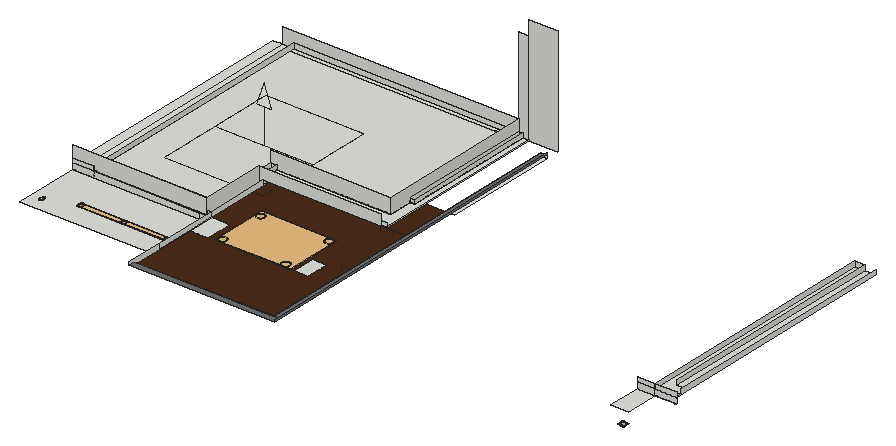
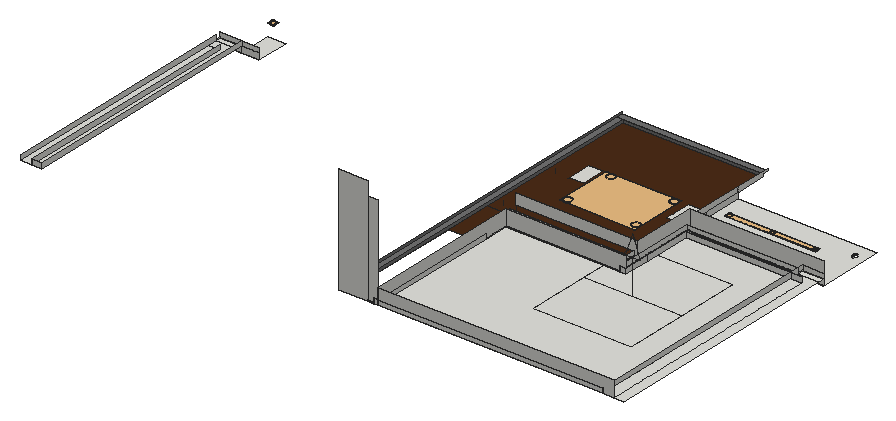
# SketchUp Ruby script. Lengths in inches.
U = 1.inch
M = Sketchup.active_model
def pt(a) = Geom::Point3d.new(a.map { |v| v * U })
def face(e, loops, mat)
  f = e.add_face(loops[0].map { |a| pt(a) })
  loops[1..].each { |l| e.add_face(l.map { |a| pt(a) }).erase! }
  f.material = f.back_material = mat if mat
  f
end
# faces: each face lists its corners as indices into pts; further lists are holes
def faces(e, pts, list, mat = nil) = list.each { |f| face(e, (f[0].is_a?(Array) ? f : [f]).map { |l| l.map { |i| pts[i] } }, mat) }
# xy, xz, yz: faces in a plane at the given z, y or x. An outline is a flat list of corners, or four numbers for a rectangle; further outlines are holes
def ring(l) = l.size == 4 ? [[l[0], l[1]], [l[2], l[1]], [l[2], l[3]], [l[0], l[3]]] : l.each_slice(2).to_a
def flat(e, list, mat, &to3) = list.each { |f| face(e, (f[0].is_a?(Array) ? f : [f]).map { |l| ring(l).map { |u, v| to3.(u, v) } }, mat) }
def xy(e, z, list, mat = nil) = flat(e, list, mat) { |x, y| [x, y, z] }
def xz(e, y, list, mat = nil) = flat(e, list, mat) { |x, z| [x, y, z] }
def yz(e, x, list, mat = nil) = flat(e, list, mat) { |y, z| [x, y, z] }
def lines(e, pts, list) = list.each { |a, b| e.add_line(pt(pts[a]), pt(pts[b])) }
# prism: a flat outline (further loops are holes) pulled along v
def prism(e, loops, v, mat = nil)
  f = face(e, loops, mat); d = Geom::Vector3d.new(v.map { |x| x * U })
  f.pushpull(f.normal.samedirection?(d) ? d.length : -d.length)
end
def box(e, o, s, mat = nil) = prism(e, [[o, [o[0] + s[0], o[1], o[2]], [o[0] + s[0], o[1] + s[1], o[2]], [o[0], o[1] + s[1], o[2]]]], [0, 0, s[2]], mat)
def at(x, y, z, deg = 0) = Geom::Transformation.translation(pt([x, y, z])) * Geom::Transformation.rotation(ORIGIN, Z_AXIS, deg.degrees)
def axes(o, x, y, z) = Geom::Transformation.new([*x, 0, *y, 0, *z, 0, *pt(o).to_a, 1])
def part(name) = M.definitions.add(name)
# library, detail: a bought-in or finely detailed component or shape, given as its bounding box
def library(name, o, s) = part(name).tap { |d| box(d.entities, o, s) }
def detail(e, o, s) = box(e.add_group.entities, o, s)
def put(e, d, t, mat = nil) = e.add_instance(d, t).tap { |i| i.material = mat if mat }
def group(e, t, mat = nil) = e.add_group.tap { |g| g.transformation = t; g.material = mat if mat }.entities
root = M.entities
M.materials.add("[Color M05]").color = [114, 114, 114]
M.materials.add("[Wood Veneer 01]").color = [76, 44, 23]
c1 = library("Group\#26",[-0.5,-0.5,-0.1],[9.125,9.125,0.2])
c2 = library("Group\#20",[-0.5,-0.5,-0.1],[139.5,7.875,0.2])
c3 = library("Group\#21",[-0.5,-0.5,-0.1],[115.36,88.99,0.2])
c4 = part("Group266\#1")
p = [[0,0,0],[0,0,-53.16],[-11.52,0,-53.16],[75.01,-97.09,0],[-75.01,-97.09,0],[75.01,97.09,0],
  [75.01,0,0],[-75.01,97.09,0],[11.52,0,-53.16],[-75.01,0,0],[0,0,-86.05]]
lines(c4.entities,p,[[0,1],[1,2],[3,4],[5,6],[7,5],[1,8],[9,0],[0,6],[8,10],[4,9],[6,3],[2,10],
  [9,7]])
c5 = part("Rectangle Light\#1")
put(c5.entities,c4,at(0,0,0))
xy(root,104.9375,[[[1172.33,1537.85,1384.3,1638.35],[1186.89,1555.5,1187.94,1555.63,1188.92,1556.04,1189.77,1556.6875,1190.41,1557.53,1190.82,1558.51,1190.96,1559.56,1190.82,1560.61,1190.41,1561.59,1189.77,1562.43,1188.92,1563.08,1187.94,1563.48,1186.89,1563.62,1185.84,1563.48,1184.86,1563.08,1184.02,1562.43,1183.375,1561.59,1182.97,1560.61,1182.83,1559.56,1182.97,1558.51,1183.375,1557.53,1184.02,1556.6875,1184.86,1556.04,1185.84,1555.63],[1234.95,1572.17,1235.84,1572.29,1236.67,1572.63,1237.38,1573.18,1237.93,1573.89,1238.27,1574.72,1238.39,1575.61,1238.27,1576.5,1237.93,1577.33,1237.38,1578.04,1236.67,1578.59,1235.84,1578.93,1234.95,1579.05,1234.06,1578.93,1233.23,1578.59,1232.52,1578.04,1231.97,1577.33,1231.63,1576.5,1231.51,1575.61,1231.63,1574.72,1231.97,1573.89,1232.52,1573.18,1233.23,1572.63,1234.06,1572.29],[1300.76,1572.17,1301.65,1572.29,1302.48,1572.63,1303.19,1573.18,1303.74,1573.89,1304.08,1574.72,1304.2,1575.61,1304.08,1576.5,1303.74,1577.33,1303.19,1578.04,1302.48,1578.59,1301.65,1578.93,1300.76,1579.05,1299.87,1578.93,1299.04,1578.59,1298.33,1578.04,1297.79,1577.33,1297.44,1576.5,1297.32,1575.61,1297.44,1574.72,1297.79,1573.89,1298.33,1573.18,1299.04,1572.63,1299.87,1572.29],[1366.57,1572.17,1367.46,1572.29,1368.29,1572.63,1369.01,1573.18,1369.55,1573.89,1369.9,1574.72,1370.01,1575.61,1369.9,1576.5,1369.55,1577.33,1369.01,1578.04,1368.29,1578.59,1367.46,1578.93,1366.57,1579.05,1365.69,1578.93,1364.86,1578.59,1364.14,1578.04,1363.6,1577.33,1363.25,1576.5,1363.14,1575.61,1363.25,1574.72,1363.6,1573.89,1364.14,1573.18,1364.86,1572.63,1365.69,1572.29]]])
xy(root,109.5,[[2037.92,1585.79,2064.92,1636.04]])
xy(root,113.8125,[[1384.3,1597.35,1411.73,1638.29],[1542.45,1597.35,1563.95,1634.91],[1172.33,1638.35,1204.64,1647.57],[1204.64,1638.35,1365.47,1647.57],[1172.33,1647.57,1204.64,1647.57,1204.64,1661.875,1187.0625,1661.875,1187.0625,2020.66,1172.33,2020.66],
  [1187.0625,1661.875,1204.64,2020.66],[1204.64,1661.875,1204.64,2013.29,1548.25,2013.29,1548.25,1775.97,1364.27,1775.97,1364.27,1661.875],[1554.73,1749.22,1563.95,2020.66],[1597.39,1824.2,1607.7,2001.02],[1204.64,2013.29,1517.39,2020.66],
  [1517.39,2013.29,1548.25,2020.66]])
xy(root,113.8125,[[[1384.3,1490.47,1384.3,1597.35,1411.73,1597.35,1411.73,1638.29,1384.3,1638.29,1384.3,1749.22,1597.39,1749.22,1597.39,1490.47],[1542.45,1597.35,1563.95,1634.91],[1525.93,1597.54,1527.48,1597.75,1528.93,1598.35,1530.17,1599.3,1531.13,1600.54,1531.73,1601.99,1531.93,1603.54,1531.73,1605.1,1531.13,1606.54,1530.17,1607.79,1528.93,1608.74,1527.48,1609.34,1525.93,1609.54,1524.38,1609.34,1522.93,1608.74,1521.6875,1607.79,1520.74,1606.54,1520.14,1605.1,1519.93,1603.54,1520.14,1601.99,1520.74,1600.54,1521.6875,1599.3,1522.93,1598.35,1524.38,1597.75],[1429.12,1597.54,1430.67,1597.75,1432.12,1598.35,1433.36,1599.3,1434.32,1600.54,1434.92,1601.99,1435.12,1603.54,1434.92,1605.1,1434.32,1606.54,1433.36,1607.79,1432.12,1608.74,1430.67,1609.34,1429.12,1609.54,1427.57,1609.34,1426.12,1608.74,1424.875,1607.79,1423.92,1606.54,1423.32,1605.1,1423.12,1603.54,1423.32,1601.99,1423.92,1600.54,1424.875,1599.3,1426.12,1598.35,1427.57,1597.75],[1429.12,1670.29,1430.67,1670.5,1432.12,1671.1,1433.36,1672.05,1434.32,1673.29,1434.92,1674.74,1435.12,1676.29,1434.92,1677.85,1434.32,1679.29,1433.36,1680.54,1432.12,1681.49,1430.67,1682.09,1429.12,1682.29,1427.57,1682.09,1426.12,1681.49,1424.875,1680.54,1423.92,1679.29,1423.32,1677.85,1423.12,1676.29,1423.32,1674.74,1423.92,1673.29,1424.875,1672.05,1426.12,1671.1,1427.57,1670.5],[1531.48,1673.53,1533.03,1673.73,1534.48,1674.33,1535.72,1675.28,1536.68,1676.53,1537.28,1677.97,1537.48,1679.53,1537.28,1681.08,1536.68,1682.53,1535.72,1683.77,1534.48,1684.72,1533.03,1685.32,1531.48,1685.53,1529.93,1685.32,1528.48,1684.72,1527.24,1683.77,1526.28,1682.53,1525.6875,1681.08,1525.48,1679.53,1525.6875,1677.97,1526.28,1676.53,1527.24,1675.28,1528.48,1674.33,1529.93,1673.73]],[1563.95,1749.22,1597.39,1824.2]],"[Wood Veneer 01]")
xy(root,115.0625,[[1204.64,1638.35,1376.89,1638.35,1376.89,1737.41,1384.3,1737.41,1384.3,1749.22,1563.95,1749.22,1563.95,2020.66,1554.73,2020.66,1554.73,1813.21,1548.25,1813.21,1548.25,1775.97,1373.95,1775.97,1373.95,1647.57,1204.64,1647.57]])
xy(root,118.1875,[[1384.3,1481.16,1607.7,1490.47],[1597.39,1490.47,1607.7,2001.02]],"[Color M05]")
xy(root,118.5,[[2064.92,1636.04,2097.23,1645.27],[2064.92,1645.27,2097.23,1645.27,2097.23,1659.57,2079.65,1659.57,2079.65,2018.36,2064.92,2018.36],[2079.65,1659.57,2097.23,2018.36]])
xz(root,1490.47,[[1384.3,113.8125,1597.39,118.1875]],"[Color M05]")
xz(root,1636.04,[[2037.92,109.5,2064.92,118.5],[2064.92,109.5,2097.23,109.625],[2064.92,109.625,2097.23,118.5],[2037.92,118.5,2064.92,126],[2064.92,118.5,2097.23,126]])
xz(root,1638.35,[[1172.33,104.8125,1204.64,104.9375],[1172.33,104.9375,1204.64,113.8125],[1204.64,104.9375,1365.47,113.8125],[1365.47,104.9375,1384.3,113.8125],[1172.33,113.8125,1204.64,121.3125],
  [1204.64,113.8125,1376.89,115.0625],[1376.89,113.8125,1384.3,121.3125],[1204.64,115.0625,1376.89,115.0625,1376.89,138.1875,1172.33,138.1875,1172.33,121.3125,1204.64,121.3125]])
xz(root,1647.57,[[1204.64,113.8125,1373.95,115.0625],[1204.64,115.0625,1373.95,121.3125]])
xz(root,1661.875,[[1187.0625,113.8125,1364.27,121.3125]])
xz(root,1737.41,[[1376.89,113.8125,1384.3,115.0625],[1376.89,115.0625,1384.3,115.0625,1384.3,121.3125,1563.95,121.3125,1563.95,138.1875,1376.89,138.1875]])
xz(root,1749.22,[[1384.3,113.8125,1554.73,115.0625],[1554.73,113.8125,1563.95,115.0625],[1384.3,115.0625,1563.95,121.3125]])
xz(root,1775.97,[[1364.27,113.8125,1373.95,121.3125],[1373.95,113.8125,1548.25,115.0625],[1373.95,115.0625,1548.25,115.0625,1548.25,138.1875,1364.27,138.1875,1364.27,121.3125,1373.95,121.3125]])
xz(root,1813.21,[[1548.25,113.8125,1554.73,115.0625],[1548.25,115.0625,1554.73,121.3125]])
xz(root,2001.02,[[1597.39,113.8125,1607.7,118.1875]])
xz(root,2018.36,[[2064.92,118.5,2079.65,126]])
xz(root,2020.66,[[1187.0625,113.8125,1187.0625,138.1875,1548.25,138.1875,1548.25,121.3125,1204.64,121.3125,1204.64,113.8125],[1204.64,113.8125,1548.25,121.3125],[1548.25,113.8125,1554.73,121.3125],[1554.73,113.8125,1563.95,115.0625],[1563.95,113.8125,1607.7,279.25],
  [1554.73,115.0625,1554.73,121.3125,1548.25,121.3125,1548.25,258.1875,1563.95,258.1875,1563.95,115.0625]])
yz(root,1204.64,[[1638.35,113.8125,1647.57,115.0625],[1647.57,113.8125,2020.66,121.3125],[1638.35,115.0625,1647.57,121.3125]])
yz(root,1364.27,[[1661.875,113.8125,1737.41,121.3125],[1737.41,113.8125,1775.97,121.3125]])
yz(root,1373.95,[[1647.57,113.8125,1775.97,115.0625],[1647.57,115.0625,1775.97,121.3125]])
yz(root,1376.89,[[1638.35,113.8125,1737.41,115.0625],[1638.35,115.0625,1737.41,138.1875]])
yz(root,1384.3,[[1537.85,104.9375,1597.35,113.8125],[1597.35,104.9375,1638.29,113.8125],[1638.29,104.9375,1638.35,113.8125],[1490.47,113.8125,1490.47,118.1875,1481.16,118.1875,1481.16,121.3125,1537.85,121.3125,1537.85,113.8125],[1537.85,113.8125,1638.35,121.3125],
  [1638.35,113.8125,1737.41,121.3125],[1737.41,113.8125,1749.22,115.0625],[1737.41,115.0625,1749.22,121.3125]])
yz(root,1548.25,[[1775.97,113.8125,1813.21,115.0625],[1813.21,113.8125,2020.66,121.3125],[1775.97,115.0625,1813.21,115.0625,1813.21,121.3125,2020.66,121.3125,2020.66,138.1875,1775.97,138.1875]])
yz(root,1554.73,[[1813.21,113.8125,2020.66,115.0625],[1813.21,115.0625,2020.66,121.3125]])
yz(root,1563.95,[[1749.22,113.8125,2020.66,115.0625]])
yz(root,1597.39,[[1490.47,113.8125,2001.02,118.1875]],"[Color M05]")
yz(root,1607.7,[[1481.16,118.1875,2001.02,121.3125]],"[Color M05]")
yz(root,2064.92,[[1636.04,118.5,2018.36,126]])
yz(root,2079.65,[[1659.57,118.5,2018.36,126]])
yz(root,2097.23,[[1636.04,118.5,1645.27,119.75],[1645.27,118.5,2018.36,126]])
p = [[1187.94,1555.63,104.9375],[1186.89,1555.5,104.9375],[1186.89,1555.5,105.875],[1187.94,1555.63,105.875],[1188.92,1556.04,104.9375],[1188.92,1556.04,105.875],
  [1189.77,1556.6875,104.9375],[1189.77,1556.6875,105.875],[1190.41,1557.53,104.9375],[1190.41,1557.53,105.875],[1190.82,1558.51,104.9375],[1190.82,1558.51,105.875],
  [1190.96,1559.56,104.9375],[1190.96,1559.56,105.875],[1190.82,1560.61,104.9375],[1190.82,1560.61,105.875],[1190.41,1561.59,104.9375],[1190.41,1561.59,105.875],
  [1189.77,1562.43,104.9375],[1189.77,1562.43,105.875],[1188.92,1563.08,104.9375],[1188.92,1563.08,105.875],[1187.94,1563.48,104.9375],[1187.94,1563.48,105.875],
  [1186.89,1563.62,104.9375],[1186.89,1563.62,105.875],[1234.95,1572.17,104.9375],[1234.06,1572.29,104.9375],[1234.06,1572.29,105.375],[1234.95,1572.17,105.375],
  [1235.84,1572.29,104.9375],[1235.84,1572.29,105.375],[1300.76,1572.17,104.9375],[1299.87,1572.29,104.9375],[1299.87,1572.29,105.375],[1300.76,1572.17,105.375],
  [1301.65,1572.29,104.9375],[1301.65,1572.29,105.375],[1366.57,1572.17,104.9375],[1365.69,1572.29,104.9375],[1365.69,1572.29,105.375],[1366.57,1572.17,105.375],
  [1367.46,1572.29,104.9375],[1367.46,1572.29,105.375],[1233.23,1572.63,104.9375],[1233.23,1572.63,105.375],[1236.67,1572.63,104.9375],[1236.67,1572.63,105.375],
  [1299.04,1572.63,104.9375],[1299.04,1572.63,105.375],[1302.48,1572.63,104.9375],[1302.48,1572.63,105.375],[1364.86,1572.63,104.9375],[1364.86,1572.63,105.375],
  [1368.29,1572.63,104.9375],[1368.29,1572.63,105.375],[1232.52,1573.18,104.9375],[1232.52,1573.18,105.375],[1237.38,1573.18,104.9375],[1237.38,1573.18,105.375],
  [1298.33,1573.18,104.9375],[1298.33,1573.18,105.375],[1303.19,1573.18,104.9375],[1303.19,1573.18,105.375],[1364.14,1573.18,104.9375],[1364.14,1573.18,105.375],
  [1369.01,1573.18,104.9375],[1369.01,1573.18,105.375],[1231.97,1573.89,104.9375],[1231.97,1573.89,105.375],[1237.93,1573.89,104.9375],[1237.93,1573.89,105.375],
  [1297.79,1573.89,104.9375],[1297.79,1573.89,105.375],[1303.74,1573.89,104.9375],[1303.74,1573.89,105.375],[1363.6,1573.89,104.9375],[1363.6,1573.89,105.375],
  [1369.55,1573.89,104.9375],[1369.55,1573.89,105.375],[1231.63,1574.72,104.9375],[1231.63,1574.72,105.375],[1238.27,1574.72,104.9375],[1238.27,1574.72,105.375],
  [1297.44,1574.72,104.9375],[1297.44,1574.72,105.375],[1304.08,1574.72,104.9375],[1304.08,1574.72,105.375],[1363.25,1574.72,104.9375],[1363.25,1574.72,105.375],
  [1369.9,1574.72,104.9375],[1369.9,1574.72,105.375],[1231.51,1575.61,104.9375],[1231.51,1575.61,105.375],[1238.39,1575.61,104.9375],[1238.39,1575.61,105.375],
  [1297.32,1575.61,104.9375],[1297.32,1575.61,105.375],[1304.2,1575.61,104.9375],[1304.2,1575.61,105.375],[1363.14,1575.61,104.9375],[1363.14,1575.61,105.375],
  [1370.01,1575.61,104.9375],[1370.01,1575.61,105.375],[1231.63,1576.5,104.9375],[1231.63,1576.5,105.375],[1238.27,1576.5,104.9375],[1238.27,1576.5,105.375],
  [1297.44,1576.5,104.9375],[1297.44,1576.5,105.375],[1304.08,1576.5,104.9375],[1304.08,1576.5,105.375],[1363.25,1576.5,104.9375],[1363.25,1576.5,105.375],
  [1369.9,1576.5,104.9375],[1369.9,1576.5,105.375],[1231.97,1577.33,104.9375],[1231.97,1577.33,105.375],[1237.93,1577.33,104.9375],[1237.93,1577.33,105.375],
  [1297.79,1577.33,104.9375],[1297.79,1577.33,105.375],[1303.74,1577.33,104.9375],[1303.74,1577.33,105.375],[1363.6,1577.33,104.9375],[1363.6,1577.33,105.375],
  [1369.55,1577.33,104.9375],[1369.55,1577.33,105.375],[1232.52,1578.04,104.9375],[1232.52,1578.04,105.375],[1237.38,1578.04,104.9375],[1237.38,1578.04,105.375],
  [1298.33,1578.04,104.9375],[1298.33,1578.04,105.375],[1303.19,1578.04,104.9375],[1303.19,1578.04,105.375],[1364.14,1578.04,104.9375],[1364.14,1578.04,105.375],
  [1369.01,1578.04,104.9375],[1369.01,1578.04,105.375],[1233.23,1578.59,104.9375],[1233.23,1578.59,105.375],[1236.67,1578.59,104.9375],[1236.67,1578.59,105.375],
  [1299.04,1578.59,104.9375],[1299.04,1578.59,105.375],[1302.48,1578.59,104.9375],[1302.48,1578.59,105.375],[1364.86,1578.59,104.9375],[1364.86,1578.59,105.375],
  [1368.29,1578.59,104.9375],[1368.29,1578.59,105.375],[1234.06,1578.93,104.9375],[1234.06,1578.93,105.375],[1235.84,1578.93,104.9375],[1235.84,1578.93,105.375],
  [1299.87,1578.93,104.9375],[1299.87,1578.93,105.375],[1301.65,1578.93,104.9375],[1301.65,1578.93,105.375],[1365.69,1578.93,104.9375],[1365.69,1578.93,105.375],
  [1367.46,1578.93,104.9375],[1367.46,1578.93,105.375],[1234.95,1579.05,104.9375],[1234.95,1579.05,105.375],[1300.76,1579.05,104.9375],[1300.76,1579.05,105.375],
  [1366.57,1579.05,104.9375],[1366.57,1579.05,105.375],[2079.48,1553.19,109.625],[2078.43,1553.33,109.625],[2078.43,1553.33,110.5625],[2079.48,1553.19,110.5625],
  [2080.53,1553.33,109.625],[2080.53,1553.33,110.5625],[2077.45,1553.73,109.625],[2077.45,1553.73,110.5625],[2081.51,1553.73,109.625],[2081.51,1553.73,110.5625],
  [2076.61,1554.38,109.625],[2076.61,1554.38,110.5625],[2082.36,1554.38,109.625],[2082.36,1554.38,110.5625],[2075.96,1555.22,109.625],[2075.96,1555.22,110.5625],
  [2083,1555.22,109.625],[2083,1555.22,110.5625],[2075.56,1556.2,109.625],[2075.56,1556.2,110.5625],[2083.41,1556.2,109.625],[2083.41,1556.2,110.5625],
  [2075.42,1557.25,109.625],[2075.42,1557.25,110.5625],[2083.55,1557.25,109.625],[2083.55,1557.25,110.5625],[2075.56,1558.3,109.625],[2075.56,1558.3,110.5625],
  [2083.41,1558.3,109.625],[2083.41,1558.3,110.5625],[2075.96,1559.28,109.625],[2075.96,1559.28,110.5625],[2083,1559.28,109.625],[2083,1559.28,110.5625],
  [2076.61,1560.125,109.625],[2076.61,1560.125,110.5625],[2082.36,1560.125,109.625],[2082.36,1560.125,110.5625],[2077.45,1560.77,109.625],[2077.45,1560.77,110.5625],
  [2081.51,1560.77,109.625],[2081.51,1560.77,110.5625],[2078.43,1561.18,109.625],[2078.43,1561.18,110.5625],[2080.53,1561.18,109.625],[2080.53,1561.18,110.5625],
  [2079.48,1561.31,109.625],[2079.48,1561.31,110.5625],[1429.12,1597.54,113.8125],[1427.57,1597.75,113.8125],[1427.57,1597.75,114.6875],[1429.12,1597.54,114.6875],
  [1430.67,1597.75,113.8125],[1430.67,1597.75,114.6875],[1525.93,1597.54,113.8125],[1524.38,1597.75,113.8125],[1524.38,1597.75,114.6875],[1525.93,1597.54,114.6875],
  [1527.48,1597.75,113.8125],[1527.48,1597.75,114.6875],[1426.12,1598.35,113.8125],[1426.12,1598.35,114.6875],[1432.12,1598.35,113.8125],[1432.12,1598.35,114.6875],
  [1522.93,1598.35,113.8125],[1522.93,1598.35,114.6875],[1528.93,1598.35,113.8125],[1528.93,1598.35,114.6875],[1424.875,1599.3,113.8125],[1424.875,1599.3,114.6875],
  [1433.36,1599.3,113.8125],[1433.36,1599.3,114.6875],[1521.6875,1599.3,113.8125],[1521.6875,1599.3,114.6875],[1530.17,1599.3,113.8125],[1530.17,1599.3,114.6875],
  [1423.92,1600.54,113.8125],[1423.92,1600.54,114.6875],[1434.32,1600.54,113.8125],[1434.32,1600.54,114.6875],[1520.74,1600.54,113.8125],[1520.74,1600.54,114.6875],
  [1531.13,1600.54,113.8125],[1531.13,1600.54,114.6875],[1423.32,1601.99,113.8125],[1423.32,1601.99,114.6875],[1434.92,1601.99,113.8125],[1434.92,1601.99,114.6875],
  [1520.14,1601.99,113.8125],[1520.14,1601.99,114.6875],[1531.73,1601.99,113.8125],[1531.73,1601.99,114.6875],[1423.12,1603.54,113.8125],[1423.12,1603.54,114.6875],
  [1435.12,1603.54,113.8125],[1435.12,1603.54,114.6875],[1519.93,1603.54,113.8125],[1519.93,1603.54,114.6875],[1531.93,1603.54,113.8125],[1531.93,1603.54,114.6875],
  [1423.32,1605.1,113.8125],[1423.32,1605.1,114.6875],[1434.92,1605.1,113.8125],[1434.92,1605.1,114.6875],[1520.14,1605.1,113.8125],[1520.14,1605.1,114.6875],
  [1531.73,1605.1,113.8125],[1531.73,1605.1,114.6875],[1423.92,1606.54,113.8125],[1423.92,1606.54,114.6875],[1434.32,1606.54,113.8125],[1434.32,1606.54,114.6875],
  [1520.74,1606.54,113.8125],[1520.74,1606.54,114.6875],[1531.13,1606.54,113.8125],[1531.13,1606.54,114.6875],[1424.875,1607.79,113.8125],[1424.875,1607.79,114.6875],
  [1433.36,1607.79,113.8125],[1433.36,1607.79,114.6875],[1521.6875,1607.79,113.8125],[1521.6875,1607.79,114.6875],[1530.17,1607.79,113.8125],[1530.17,1607.79,114.6875],
  [1426.12,1608.74,113.8125],[1426.12,1608.74,114.6875],[1432.12,1608.74,113.8125],[1432.12,1608.74,114.6875],[1522.93,1608.74,113.8125],[1522.93,1608.74,114.6875],
  [1528.93,1608.74,113.8125],[1528.93,1608.74,114.6875],[1427.57,1609.34,113.8125],[1427.57,1609.34,114.6875],[1430.67,1609.34,113.8125],[1430.67,1609.34,114.6875],
  [1524.38,1609.34,113.8125],[1524.38,1609.34,114.6875],[1527.48,1609.34,113.8125],[1527.48,1609.34,114.6875],[1429.12,1609.54,113.8125],[1429.12,1609.54,114.6875],
  [1525.93,1609.54,113.8125],[1525.93,1609.54,114.6875],[1429.12,1670.29,113.8125],[1427.57,1670.5,113.8125],[1427.57,1670.5,114.6875],[1429.12,1670.29,114.6875],
  [1430.67,1670.5,113.8125],[1430.67,1670.5,114.6875],[1426.12,1671.1,113.8125],[1426.12,1671.1,114.6875],[1432.12,1671.1,113.8125],[1432.12,1671.1,114.6875],
  [1424.875,1672.05,113.8125],[1424.875,1672.05,114.6875],[1433.36,1672.05,113.8125],[1433.36,1672.05,114.6875],[1423.92,1673.29,113.8125],[1423.92,1673.29,114.6875],
  [1434.32,1673.29,113.8125],[1434.32,1673.29,114.6875],[1423.32,1674.74,113.8125],[1423.32,1674.74,114.6875],[1434.92,1674.74,113.8125],[1434.92,1674.74,114.6875],
  [1531.48,1673.53,113.8125],[1529.93,1673.73,113.8125],[1529.93,1673.73,114.6875],[1531.48,1673.53,114.6875],[1533.03,1673.73,113.8125],[1533.03,1673.73,114.6875],
  [1528.48,1674.33,113.8125],[1528.48,1674.33,114.6875],[1534.48,1674.33,113.8125],[1534.48,1674.33,114.6875],[1527.24,1675.28,113.8125],[1527.24,1675.28,114.6875],
  [1535.72,1675.28,113.8125],[1535.72,1675.28,114.6875],[1423.12,1676.29,113.8125],[1423.12,1676.29,114.6875],[1435.12,1676.29,113.8125],[1435.12,1676.29,114.6875],
  [1526.28,1676.53,113.8125],[1526.28,1676.53,114.6875],[1536.68,1676.53,113.8125],[1536.68,1676.53,114.6875],[1423.32,1677.85,113.8125],[1423.32,1677.85,114.6875],
  [1434.92,1677.85,113.8125],[1434.92,1677.85,114.6875],[1525.6875,1677.97,113.8125],[1525.6875,1677.97,114.6875],[1537.28,1677.97,113.8125],[1537.28,1677.97,114.6875],
  [1423.92,1679.29,113.8125],[1423.92,1679.29,114.6875],[1434.32,1679.29,113.8125],[1434.32,1679.29,114.6875],[1525.48,1679.53,113.8125],[1525.48,1679.53,114.6875],
  [1537.48,1679.53,113.8125],[1537.48,1679.53,114.6875],[1424.875,1680.54,113.8125],[1424.875,1680.54,114.6875],[1433.36,1680.54,113.8125],[1433.36,1680.54,114.6875],
  [1525.6875,1681.08,113.8125],[1525.6875,1681.08,114.6875],[1537.28,1681.08,113.8125],[1537.28,1681.08,114.6875],[1426.12,1681.49,113.8125],[1426.12,1681.49,114.6875],
  [1432.12,1681.49,113.8125],[1432.12,1681.49,114.6875],[1526.28,1682.53,113.8125],[1526.28,1682.53,114.6875],[1536.68,1682.53,113.8125],[1536.68,1682.53,114.6875],
  [1427.57,1682.09,113.8125],[1427.57,1682.09,114.6875],[1430.67,1682.09,113.8125],[1430.67,1682.09,114.6875],[1429.12,1682.29,113.8125],[1429.12,1682.29,114.6875],
  [1527.24,1683.77,113.8125],[1527.24,1683.77,114.6875],[1535.72,1683.77,113.8125],[1535.72,1683.77,114.6875],[1528.48,1684.72,113.8125],[1528.48,1684.72,114.6875],
  [1534.48,1684.72,113.8125],[1534.48,1684.72,114.6875],[1529.93,1685.32,113.8125],[1529.93,1685.32,114.6875],[1533.03,1685.32,113.8125],[1533.03,1685.32,114.6875],
  [1531.48,1685.53,113.8125],[1531.48,1685.53,114.6875],[1583.39,1638.35,113.8125],[1583.39,1638.29,113.8125],[1583.39,1737.41,121.3125],[1583.39,1737.41,113.8125],
  [1563.95,1737.41,121.3125],[1563.95,1737.41,113.8125],[1563.95,1638.29,113.8125],[1563.95,1634.91,113.8125],[1583.39,1638.35,121.3125]]
faces(root,p,[[0,1,2,3],[4,0,3,5],[6,4,5,7],[8,6,7,9],[10,8,9,11],[12,10,11,13],[14,12,13,15],[16,14,15,17],
  [18,16,17,19],[20,18,19,21],[22,20,21,23],[24,22,23,25],[26,27,28,29],[30,26,29,31],[32,33,34,35],[36,32,35,37],
  [38,39,40,41],[42,38,41,43],[27,44,45,28],[46,30,31,47],[33,48,49,34],[50,36,37,51],[39,52,53,40],[54,42,43,55],
  [44,56,57,45],[58,46,47,59],[48,60,61,49],[62,50,51,63],[52,64,65,53],[66,54,55,67],[56,68,69,57],[70,58,59,71],
  [60,72,73,61],[74,62,63,75],[64,76,77,65],[78,66,67,79],[68,80,81,69],[82,70,71,83],[72,84,85,73],[86,74,75,87],
  [76,88,89,77],[90,78,79,91],[80,92,93,81],[94,82,83,95],[84,96,97,85],[98,86,87,99],[88,100,101,89],[102,90,91,103],
  [92,104,105,93],[106,94,95,107],[96,108,109,97],[110,98,99,111],[100,112,113,101],[114,102,103,115],[104,116,117,105],[118,106,107,119],
  [108,120,121,109],[122,110,111,123],[112,124,125,113],[126,114,115,127],[116,128,129,117],[130,118,119,131],[120,132,133,121],[134,122,123,135],
  [124,136,137,125],[138,126,127,139],[128,140,141,129],[142,130,131,143],[132,144,145,133],[146,134,135,147],[136,148,149,137],[150,138,139,151],
  [140,152,153,141],[154,142,143,155],[144,156,157,145],[158,146,147,159],[148,160,161,149],[162,150,151,163],[152,164,165,153],[164,154,155,165],
  [156,166,167,157],[166,158,159,167],[160,168,169,161],[168,162,163,169],[170,171,172,173],[174,170,173,175],[171,176,177,172],[178,174,175,179],
  [176,180,181,177],[182,178,179,183],[180,184,185,181],[186,182,183,187],[184,188,189,185],[190,186,187,191],[188,192,193,189],[194,190,191,195],
  [192,196,197,193],[198,194,195,199],[196,200,201,197],[202,198,199,203],[200,204,205,201],[206,202,203,207],[204,208,209,205],[210,206,207,211],
  [208,212,213,209],[214,210,211,215],[212,216,217,213],[216,214,215,217]])
faces(root,p,[[218,219,220,221],[222,218,221,223],[224,225,226,227],[228,224,227,229],[219,230,231,220],[232,222,223,233],[225,234,235,226],[236,228,229,237],
  [230,238,239,231],[240,232,233,241],[234,242,243,235],[244,236,237,245],[238,246,247,239],[248,240,241,249],[242,250,251,243],[252,244,245,253],
  [246,254,255,247],[256,248,249,257],[250,258,259,251],[260,252,253,261],[254,262,263,255],[264,256,257,265],[258,266,267,259],[268,260,261,269],
  [262,270,271,263],[272,264,265,273],[266,274,275,267],[276,268,269,277],[270,278,279,271],[280,272,273,281],[274,282,283,275],[284,276,277,285],
  [278,286,287,279],[288,280,281,289],[282,290,291,283],[292,284,285,293],[286,294,295,287],[296,288,289,297],[290,298,299,291],[300,292,293,301],
  [294,302,303,295],[304,296,297,305],[298,306,307,299],[308,300,301,309],[302,310,311,303],[310,304,305,311],[306,312,313,307],[312,308,309,313],
  [314,315,316,317],[318,314,317,319],[315,320,321,316],[322,318,319,323],[320,324,325,321],[326,322,323,327],[324,328,329,325],[330,326,327,331],
  [328,332,333,329],[334,330,331,335],[336,337,338,339],[340,336,339,341],[337,342,343,338],[344,340,341,345],[342,346,347,343],[348,344,345,349],
  [332,350,351,333],[352,334,335,353],[346,354,355,347],[356,348,349,357],[350,358,359,351],[360,352,353,361],[354,362,363,355],[364,356,357,365],
  [358,366,367,359],[368,360,361,369],[362,370,371,363],[372,364,365,373],[366,374,375,367],[376,368,369,377],[370,378,379,371],[380,372,373,381],
  [374,382,383,375],[384,376,377,385],[378,386,387,379],[388,380,381,389],[382,390,391,383],[392,384,385,393],[390,394,395,391],[394,392,393,395],
  [386,396,397,387],[398,388,389,399],[396,400,401,397],[402,398,399,403],[400,404,405,401],[406,402,403,407],[404,408,409,405],[408,406,407,409]],"[Wood Veneer 01]")
lines(root,p,[[410,411],[412,413],[414,415],[416,417],[410,418]])
put(root,c1,at(2075.42,1553.19,110.5625))
put(root,c2,at(1231.51,1572.17,105.375))
put(root,c3,at(1423.12,1597.54,114.6875))
put(root,c5,axes([1323.92,1814.08,113.82],[1,0,0],[0,1,0],[0,0,-1]))
